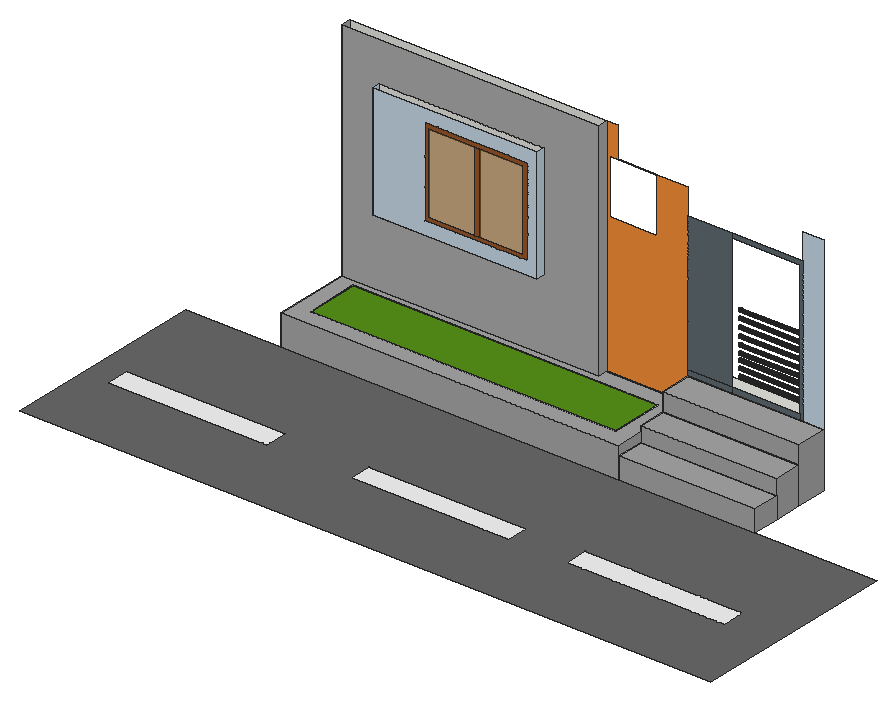
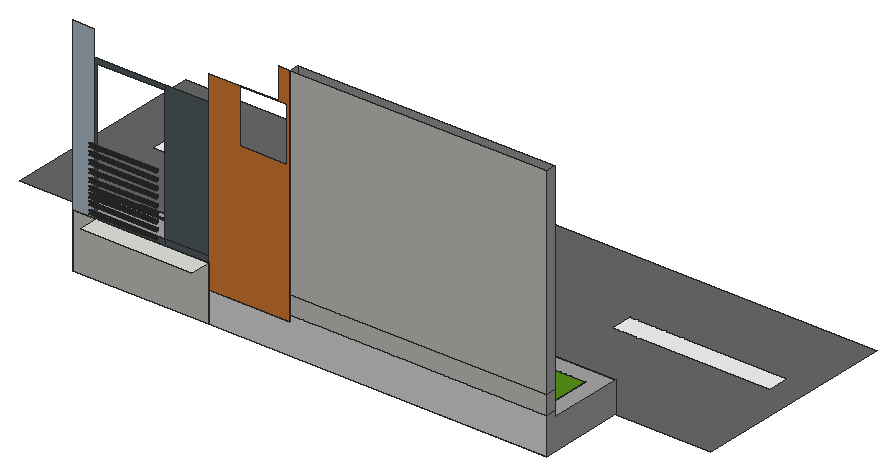
# SketchUp Ruby script. Lengths in inches.
U = 1.inch
M = Sketchup.active_model
def pt(a) = Geom::Point3d.new(a.map { |v| v * U })
def face(e, loops, mat)
  f = e.add_face(loops[0].map { |a| pt(a) })
  loops[1..].each { |l| e.add_face(l.map { |a| pt(a) }).erase! }
  f.material = f.back_material = mat if mat
  f
end
# faces: each face lists its corners as indices into pts; further lists are holes
def faces(e, pts, list, mat = nil) = list.each { |f| face(e, (f[0].is_a?(Array) ? f : [f]).map { |l| l.map { |i| pts[i] } }, mat) }
# xy, xz, yz: faces in a plane at the given z, y or x. An outline is a flat list of corners, or four numbers for a rectangle; further outlines are holes
def ring(l) = l.size == 4 ? [[l[0], l[1]], [l[2], l[1]], [l[2], l[3]], [l[0], l[3]]] : l.each_slice(2).to_a
def flat(e, list, mat, &to3) = list.each { |f| face(e, (f[0].is_a?(Array) ? f : [f]).map { |l| ring(l).map { |u, v| to3.(u, v) } }, mat) }
def xy(e, z, list, mat = nil) = flat(e, list, mat) { |x, y| [x, y, z] }
def xz(e, y, list, mat = nil) = flat(e, list, mat) { |x, z| [x, y, z] }
def yz(e, x, list, mat = nil) = flat(e, list, mat) { |y, z| [x, y, z] }
def lines(e, pts, list) = list.each { |a, b| e.add_line(pt(pts[a]), pt(pts[b])) }
# prism: a flat outline (further loops are holes) pulled along v
def prism(e, loops, v, mat = nil)
  f = face(e, loops, mat); d = Geom::Vector3d.new(v.map { |x| x * U })
  f.pushpull(f.normal.samedirection?(d) ? d.length : -d.length)
end
def box(e, o, s, mat = nil) = prism(e, [[o, [o[0] + s[0], o[1], o[2]], [o[0] + s[0], o[1] + s[1], o[2]], [o[0], o[1] + s[1], o[2]]]], [0, 0, s[2]], mat)
def at(x, y, z, deg = 0) = Geom::Transformation.translation(pt([x, y, z])) * Geom::Transformation.rotation(ORIGIN, Z_AXIS, deg.degrees)
def axes(o, x, y, z) = Geom::Transformation.new([*x, 0, *y, 0, *z, 0, *pt(o).to_a, 1])
def part(name) = M.definitions.add(name)
# library, detail: a bought-in or finely detailed component or shape, given as its bounding box
def library(name, o, s) = part(name).tap { |d| box(d.entities, o, s) }
def detail(e, o, s) = box(e.add_group.entities, o, s)
def put(e, d, t, mat = nil) = e.add_instance(d, t).tap { |i| i.material = mat if mat }
def group(e, t, mat = nil) = e.add_group.tap { |g| g.transformation = t; g.material = mat if mat }.entities
root = M.entities
M.materials.add("[0129_WhiteSmoke]").color = [245, 245, 245]
M.materials.add("[0134_DimGray]").color = [105, 105, 105]
M.materials.add("[Cladding Siding Tan]").color = [242, 141, 55]
M.materials.add("[Color M03]").color = [170, 170, 170]
M.materials.add("[Formica Laminate Dark]").color = [50, 53, 60]
M.materials.add("[Formica Speckled Grey]").color = [94, 105, 111]
M.materials.add("[Quartz Light Grey]").color = [251, 251, 252]
M.materials.add("[Stone Vein Gray]").color = [166, 165, 165]
M.materials.add("[Terrazzo Light Blue]").color = [196, 214, 227]
M.materials.add("[Translucent Glass Gray]").color = [175, 113, 36]
M.materials["[Translucent Glass Gray]"].alpha = 0.5
M.materials.add("[Vegetation Honey Locust]").color = [86, 145, 25]
M.materials.add("[Wood Cherry Original]1").color = [152, 86, 42]
xy(root,0,[[259.37,123.47,340.49,139.92],[259.37,139.92,340.49,156.38],[259.37,156.38,340.49,175.06]])
xy(root,0,[[15.62,46.64,110.16,60.39],[160.18,46.64,254.72,60.39],[289.56,46.64,384.09,60.39]],"[0129_WhiteSmoke]")
xy(root,0,[[[0,0,413.34,123.47],[15.62,46.64,110.16,60.39],[160.18,46.64,254.72,60.39],[289.56,46.64,384.09,60.39]]],"[0134_DimGray]")
xy(root,0,[[[57.16,123.47,259.37,175.06],[67.03,133.34,249.49,165.18]],[67.03,133.34,249.49,165.18]],"[Quartz Light Grey]")
xy(root,12.75,[[259.37,123.47,340.49,139.92]],"[Stone Vein Gray]")
xy(root,18.25,[[67.03,133.34,249.49,165.18]],"[Vegetation Honey Locust]")
xy(root,18.375,[[[57.16,123.47,259.37,123.47,259.37,175.06,210.68,175.06,210.68,169,57.16,169],[67.03,133.34,249.49,165.18]]],"[Stone Vein Gray]")
xy(root,21.8125,[[259.37,139.92,340.49,156.38]],"[Stone Vein Gray]")
xy(root,32.8125,[[259.37,175.06,326.14,187.5]])
xy(root,32.8125,[[259.37,156.38,340.49,175.06]],"[Stone Vein Gray]")
xy(root,60.95,[[79.41,164.37,177.78,169]],"[Terrazzo Light Blue]")
xz(root,123.47,[[57.16,0,259.37,18.375],[259.37,0,340.49,12.75]],"[Stone Vein Gray]")
xz(root,133.34,[[67.03,0,249.49,18.25]],"[Quartz Light Grey]")
xz(root,133.34,[[67.03,18.25,249.49,18.375]],"[Stone Vein Gray]")
xz(root,139.92,[[259.37,0,340.49,12.75]])
xz(root,139.92,[[259.37,12.75,340.49,21.8125]],"[Stone Vein Gray]")
xz(root,156.38,[[259.37,0,340.49,21.8125]])
xz(root,156.38,[[259.37,21.8125,340.49,32.8125]],"[Stone Vein Gray]")
xz(root,164.37,[[[79.41,60.95,177.78,129.14],[110.42,68.5625,171.92,121.4375]]],"[Terrazzo Light Blue]")
xz(root,164.37,[[113.02,71.16,140.64,118.84],[143.53,71.16,169.32,118.84]],"[Translucent Glass Gray]")
xz(root,164.37,[[[110.42,68.5625,171.92,121.4375],[113.02,71.16,169.32,118.84]],[140.64,71.16,143.53,118.84]],"[Wood Cherry Original]1")
xz(root,165.18,[[67.03,0,249.49,18.25]],"[Quartz Light Grey]")
xz(root,165.18,[[67.03,18.25,249.49,18.375]],"[Stone Vein Gray]")
xz(root,169,[[79.41,60.95,177.78,129.14]])
xz(root,169,[[[57.16,18.375,210.68,152.8125],[79.41,60.95,177.78,129.14]]],"[Color M03]")
xz(root,175.06,[[259.37,0,340.49,32.8125],[57.16,21.8125,210.68,32.8125],[57.16,32.8125,210.68,152.8125]])
xz(root,175.06,[[[210.68,18.375,259.37,18.375,259.37,134.25,217.34,134.25,217.34,152.8125,210.68,152.8125],[212.44,101.78,240.69,134.22]]],"[Cladding Siding Tan]")
xz(root,175.06,[[259.37,32.8125,285.76,36.375],[285.76,32.8125,326.14,36.375],[326.14,32.8125,328.05,32.8125,328.05,119,285.76,119,285.76,116.03,326.14,116.03],[259.37,36.375,285.76,119]],"[Formica Speckled Grey]")
xz(root,175.06,[[57.16,0,259.37,0,259.37,18.375,210.68,18.375,210.68,21.8125,57.16,21.8125]],"[Quartz Light Grey]")
xz(root,175.06,[[328.05,32.8125,340.49,134.25]],"[Terrazzo Light Blue]")
yz(root,57.16,[[169,21.8125,175.06,32.8125],[169,32.8125,175.06,152.8125]],"[Color M03]")
yz(root,57.16,[[123.47,0,123.47,18.375,169,18.375,169,21.8125,175.06,21.8125,175.06,0]],"[Stone Vein Gray]")
yz(root,67.03,[[133.34,0,165.18,18.25]],"[Quartz Light Grey]")
yz(root,67.03,[[133.34,18.25,165.18,18.375]],"[Stone Vein Gray]")
yz(root,79.41,[[164.37,60.95,169,129.14]],"[Terrazzo Light Blue]")
yz(root,177.78,[[164.37,60.95,169,129.14]],"[Terrazzo Light Blue]")
yz(root,210.68,[[169,18.375,175.06,152.8125]],"[Color M03]")
yz(root,249.49,[[133.34,0,139.92,18.25],[139.92,0,156.38,18.25],[156.38,0,165.18,18.25]],"[Quartz Light Grey]")
yz(root,249.49,[[133.34,18.25,139.92,18.375],[139.92,18.25,156.38,18.375],[156.38,18.25,165.18,18.375]],"[Stone Vein Gray]")
yz(root,259.37,[[123.47,0,139.92,12.75]])
yz(root,259.37,[[139.92,0,156.38,18.375],[156.38,0,175.06,18.375]],"[Quartz Light Grey]")
yz(root,259.37,[[123.47,12.75,139.92,18.375],[139.92,18.375,156.38,21.8125],[156.38,18.375,175.06,32.8125]],"[Stone Vein Gray]")
yz(root,340.49,[[123.47,0,139.92,12.75],[139.92,0,156.38,21.8125],[156.38,0,175.06,32.8125]],"[Stone Vein Gray]")
p = [[285.76,180.85,38.48],[285.76,181.12,38.37],[326.14,181.12,38.37],[326.14,180.85,38.48],[285.76,180.62,38.66],[326.14,180.62,38.66],
  [285.76,180.4375,38.9],[326.14,180.4375,38.9],[285.76,180.33,39.17],[326.14,180.33,39.17],[285.76,180.29,39.46],[326.14,180.29,39.46],
  [285.76,180.33,39.75],[326.14,180.33,39.75],[285.76,180.4375,40.02],[326.14,180.4375,40.02],[285.76,180.62,40.25],[326.14,180.62,40.25],
  [285.76,180.85,40.43],[326.14,180.85,40.43],[285.76,181.12,40.55],[326.14,181.12,40.55],[285.76,180.72,42.95],[285.76,180.99,42.84],
  [326.14,180.99,42.84],[326.14,180.72,42.95],[285.76,180.49,43.125],[326.14,180.49,43.125],[285.76,180.31,43.36],[326.14,180.31,43.36],
  [285.76,180.2,43.63],[326.14,180.2,43.63],[285.76,180.16,43.92],[326.14,180.16,43.92],[285.76,180.2,44.21],[326.14,180.2,44.21],
  [285.76,180.31,44.48],[326.14,180.31,44.48],[285.76,180.49,44.72],[326.14,180.49,44.72],[285.76,180.72,44.9],[326.14,180.72,44.9],
  [285.76,180.99,45.01],[326.14,180.99,45.01],[285.76,180.96,47.07],[285.76,181.25,47.03],[326.14,181.25,47.03],[326.14,180.96,47.07],
  [285.76,180.6875,47.18],[326.14,180.6875,47.18],[285.76,180.45,47.36],[326.14,180.45,47.36],[285.76,180.28,47.59],[326.14,180.28,47.59],
  [285.76,180.16,47.86],[326.14,180.16,47.86],[285.76,180.125,48.15],[326.14,180.125,48.15],[285.76,180.16,48.44],[326.14,180.16,48.44],
  [285.76,180.28,48.72],[326.14,180.28,48.72],[285.76,180.45,48.95],[326.14,180.45,48.95],[285.76,180.6875,49.13],[326.14,180.6875,49.13],
  [285.76,180.96,49.24],[326.14,180.96,49.24],[285.76,181.25,49.28],[326.14,181.25,49.28],[285.76,180.6875,51.24],[285.76,180.96,51.13],
  [326.14,180.96,51.13],[326.14,180.6875,51.24],[285.76,180.45,51.42],[326.14,180.45,51.42],[285.76,180.28,51.65],[326.14,180.28,51.65],
  [285.76,180.16,51.92],[326.14,180.16,51.92],[285.76,180.125,52.22],[326.14,180.125,52.22],[285.76,180.16,52.51],[326.14,180.16,52.51],
  [285.76,180.28,52.78],[326.14,180.28,52.78],[285.76,180.45,53.01],[326.14,180.45,53.01],[285.76,180.6875,53.19],[326.14,180.6875,53.19],
  [285.76,180.96,53.3],[326.14,180.96,53.3],[285.76,180.6875,55.62],[285.76,180.96,55.5],[326.14,180.96,55.5],[326.14,180.6875,55.62],
  [285.76,180.45,55.8],[326.14,180.45,55.8],[285.76,180.28,56.03],[326.14,180.28,56.03],[285.76,180.16,56.3],[326.14,180.16,56.3],
  [285.76,180.125,56.59],[326.14,180.125,56.59],[285.76,180.16,56.88],[326.14,180.16,56.88],[285.76,180.28,57.15],[326.14,180.28,57.15],
  [285.76,180.45,57.39],[326.14,180.45,57.39],[285.76,180.6875,57.57],[326.14,180.6875,57.57],[285.76,180.96,57.68],[326.14,180.96,57.68],
  [285.76,180.6875,60.3],[285.76,180.96,60.19],[326.14,180.96,60.19],[326.14,180.6875,60.3],[285.76,180.45,60.48],[326.14,180.45,60.48],
  [285.76,180.28,60.72],[326.14,180.28,60.72],[285.76,180.16,60.99],[326.14,180.16,60.99],[285.76,180.125,61.28],[326.14,180.125,61.28],
  [285.76,180.16,61.57],[326.14,180.16,61.57],[285.76,180.28,61.84],[326.14,180.28,61.84],[285.76,180.45,62.07],[326.14,180.45,62.07],
  [285.76,180.6875,62.25],[326.14,180.6875,62.25],[285.76,180.96,62.37],[326.14,180.96,62.37],[285.76,180.6875,64.99],[285.76,180.96,64.88],
  [326.14,180.96,64.88],[326.14,180.6875,64.99],[285.76,180.45,65.17],[326.14,180.45,65.17],[285.76,180.28,65.4],[326.14,180.28,65.4],
  [285.76,180.16,65.67],[326.14,180.16,65.67],[285.76,180.125,65.97],[326.14,180.125,65.97],[285.76,180.16,66.26],[326.14,180.16,66.26],
  [285.76,180.28,66.53],[326.14,180.28,66.53],[285.76,180.45,66.76],[326.14,180.45,66.76],[285.76,180.6875,66.94],[326.14,180.6875,66.94],
  [285.76,180.96,67.05],[326.14,180.96,67.05],[285.76,180.6875,69.68],[285.76,180.96,69.57],[326.14,180.96,69.57],[326.14,180.6875,69.68],
  [285.76,180.45,69.86],[326.14,180.45,69.86],[285.76,180.28,70.09],[326.14,180.28,70.09],[285.76,180.16,70.36],[326.14,180.16,70.36],
  [285.76,180.125,70.65],[326.14,180.125,70.65],[285.76,180.16,70.94],[326.14,180.16,70.94],[285.76,180.28,71.22],[326.14,180.28,71.22],
  [285.76,180.45,71.45],[326.14,180.45,71.45],[285.76,180.6875,71.63],[326.14,180.6875,71.63],[285.76,180.96,71.74],[326.14,180.96,71.74],
  [285.76,180.6875,74.37],[285.76,180.96,74.25],[326.14,180.96,74.25],[326.14,180.6875,74.37],[285.76,180.45,74.55],[326.14,180.45,74.55],
  [285.76,180.28,74.78],[326.14,180.28,74.78],[285.76,180.16,75.05],[326.14,180.16,75.05],[285.76,180.125,75.34],[326.14,180.125,75.34],
  [285.76,180.16,75.63],[326.14,180.16,75.63],[285.76,180.28,75.9],[326.14,180.28,75.9],[285.76,180.45,76.14],[326.14,180.45,76.14],
  [285.76,180.6875,76.32],[326.14,180.6875,76.32],[285.76,180.96,76.43],[326.14,180.96,76.43]]
faces(root,p,[[0,1,2,3],[4,0,3,5],[6,4,5,7],[8,6,7,9],[10,8,9,11],[12,10,11,13],[14,12,13,15],[16,14,15,17],
  [18,16,17,19],[20,18,19,21],[22,23,24,25],[26,22,25,27],[28,26,27,29],[30,28,29,31],[32,30,31,33],[34,32,33,35],
  [36,34,35,37],[38,36,37,39],[40,38,39,41],[42,40,41,43],[44,45,46,47],[48,44,47,49],[50,48,49,51],[52,50,51,53],
  [54,52,53,55],[56,54,55,57],[58,56,57,59],[60,58,59,61],[62,60,61,63],[64,62,63,65],[66,64,65,67],[68,66,67,69],
  [70,71,72,73],[74,70,73,75],[76,74,75,77],[78,76,77,79],[80,78,79,81],[82,80,81,83],[84,82,83,85],[86,84,85,87],
  [88,86,87,89],[90,88,89,91],[92,93,94,95],[96,92,95,97],[98,96,97,99],[100,98,99,101],[102,100,101,103],[104,102,103,105],
  [106,104,105,107],[108,106,107,109],[110,108,109,111],[112,110,111,113],[114,115,116,117],[118,114,117,119],[120,118,119,121],[122,120,121,123],
  [124,122,123,125],[126,124,125,127],[128,126,127,129],[130,128,129,131],[132,130,131,133],[134,132,133,135],[136,137,138,139],[140,136,139,141],
  [142,140,141,143],[144,142,143,145],[146,144,145,147],[148,146,147,149],[150,148,149,151],[152,150,151,153],[154,152,153,155],[156,154,155,157],
  [158,159,160,161],[162,158,161,163],[164,162,163,165],[166,164,165,167],[168,166,167,169],[170,168,169,171],[172,170,171,173],[174,172,173,175],
  [176,174,175,177],[178,176,177,179],[180,181,182,183],[184,180,183,185],[186,184,185,187],[188,186,187,189],[190,188,189,191],[192,190,191,193],
  [194,192,193,195],[196,194,195,197],[198,196,197,199],[200,198,199,201]],"[Formica Laminate Dark]")
